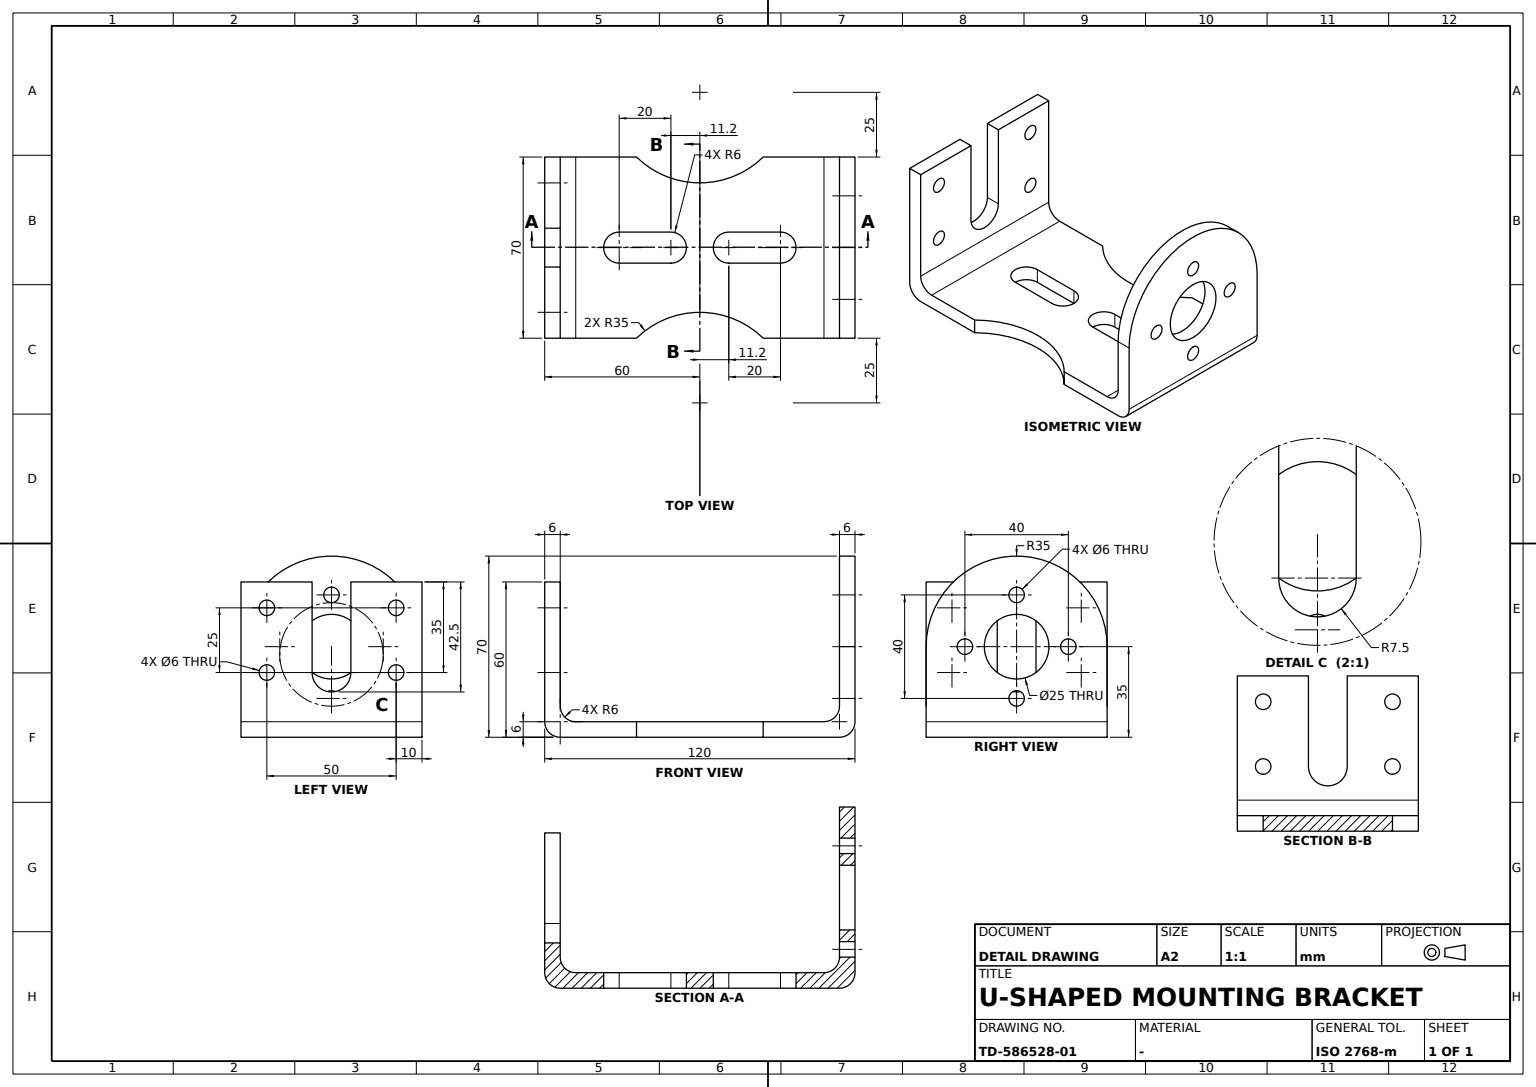
ISO-10303-21;
HEADER;
FILE_DESCRIPTION((''),'2;1');
FILE_NAME('','',(''),(''),'','','');
FILE_SCHEMA(('AUTOMOTIVE_DESIGN'));
ENDSEC;
DATA;
#1=APPLICATION_CONTEXT('');
#2=PRODUCT_CONTEXT('',#1,'mechanical');
#3=PRODUCT('','','',(#2));
#4=PRODUCT_DEFINITION_FORMATION('','',#3);
#5=PRODUCT_DEFINITION_CONTEXT('',#1,'design');
#6=PRODUCT_DEFINITION('','',#4,#5);
#7=PRODUCT_DEFINITION_SHAPE('','',#6);
#8=(LENGTH_UNIT()NAMED_UNIT(*)SI_UNIT(.MILLI.,.METRE.));
#9=(NAMED_UNIT(*)PLANE_ANGLE_UNIT()SI_UNIT($,.RADIAN.));
#10=(NAMED_UNIT(*)SI_UNIT($,.STERADIAN.)SOLID_ANGLE_UNIT());
#11=UNCERTAINTY_MEASURE_WITH_UNIT(LENGTH_MEASURE(0.005),#8,'distance_accuracy_value','');
#12=(GEOMETRIC_REPRESENTATION_CONTEXT(3)GLOBAL_UNCERTAINTY_ASSIGNED_CONTEXT((#11))GLOBAL_UNIT_ASSIGNED_CONTEXT((#8,#9,#10))REPRESENTATION_CONTEXT('',''));
#13=CARTESIAN_POINT('',(70.,35.505103,0.));
#14=VERTEX_POINT('',#13);
#15=CARTESIAN_POINT('',(70.,35.505103,6.));
#16=VERTEX_POINT('',#15);
#17=DIRECTION('',(0.,0.,1.));
#18=VECTOR('',#17,1000.);
#19=LINE('',#13,#18);
#20=EDGE_CURVE('',#14,#16,#19,.T.);
#21=ORIENTED_EDGE('',*,*,#20,.F.);
#22=CARTESIAN_POINT('',(70.,84.494897,0.));
#23=VERTEX_POINT('',#22);
#24=CARTESIAN_POINT('',(95.,60.,0.));
#25=DIRECTION('',(1.,0.,0.));
#26=AXIS2_PLACEMENT_3D('',#24,#17,#25);
#27=CIRCLE('',#26,35.);
#28=EDGE_CURVE('',#23,#14,#27,.T.);
#29=ORIENTED_EDGE('',*,*,#28,.F.);
#30=CARTESIAN_POINT('',(70.,84.494897,6.));
#31=VERTEX_POINT('',#30);
#32=LINE('',#22,#18);
#33=EDGE_CURVE('',#23,#31,#32,.T.);
#34=ORIENTED_EDGE('',*,*,#33,.T.);
#35=CARTESIAN_POINT('',(95.,60.,6.));
#36=AXIS2_PLACEMENT_3D('',#35,#17,#25);
#37=CIRCLE('',#36,35.);
#38=EDGE_CURVE('',#31,#16,#37,.T.);
#39=ORIENTED_EDGE('',*,*,#38,.T.);
#40=EDGE_LOOP('',(#21,#29,#34,#39));
#41=FACE_BOUND('',#40,.T.);
#42=CARTESIAN_POINT('',(95.,60.,3.));
#43=DIRECTION('',(0.,1.,0.));
#44=AXIS2_PLACEMENT_3D('',#42,#17,#43);
#45=CYLINDRICAL_SURFACE('',#44,35.);
#46=ADVANCED_FACE('',(#41),#45,.F.);
#47=CARTESIAN_POINT('',(27.5,6.,25.));
#48=VERTEX_POINT('',#47);
#49=CARTESIAN_POINT('',(42.5,6.,25.));
#50=VERTEX_POINT('',#49);
#51=CARTESIAN_POINT('',(35.,6.,25.));
#52=DIRECTION('',(0.,-1.,0.));
#53=DIRECTION('',(0.,0.,-1.));
#54=AXIS2_PLACEMENT_3D('',#51,#52,#53);
#55=CIRCLE('',#54,7.5);
#56=EDGE_CURVE('',#48,#50,#55,.T.);
#57=ORIENTED_EDGE('',*,*,#56,.F.);
#58=CARTESIAN_POINT('',(27.5,0.,25.));
#59=VERTEX_POINT('',#58);
#60=CARTESIAN_POINT('',(27.5,3.,25.));
#61=VECTOR('',#52,1000.);
#62=LINE('',#60,#61);
#63=EDGE_CURVE('',#59,#48,#62,.F.);
#64=ORIENTED_EDGE('',*,*,#63,.F.);
#65=CARTESIAN_POINT('',(42.5,0.,25.));
#66=VERTEX_POINT('',#65);
#67=CARTESIAN_POINT('',(35.,0.,25.));
#68=AXIS2_PLACEMENT_3D('',#67,#52,#53);
#69=CIRCLE('',#68,7.5);
#70=EDGE_CURVE('',#59,#66,#69,.T.);
#71=ORIENTED_EDGE('',*,*,#70,.T.);
#72=CARTESIAN_POINT('',(42.5,3.,25.));
#73=LINE('',#72,#61);
#74=EDGE_CURVE('',#66,#50,#73,.F.);
#75=ORIENTED_EDGE('',*,*,#74,.T.);
#76=EDGE_LOOP('',(#57,#64,#71,#75));
#77=FACE_BOUND('',#76,.T.);
#78=CARTESIAN_POINT('',(35.,3.,25.));
#79=AXIS2_PLACEMENT_3D('',#78,#52,#25);
#80=CYLINDRICAL_SURFACE('',#79,7.5);
#81=ADVANCED_FACE('',(#77),#80,.F.);
#82=CARTESIAN_POINT('',(70.,6.,0.));
#83=VERTEX_POINT('',#82);
#84=CARTESIAN_POINT('',(70.,0.,0.));
#85=LINE('',#84,#61);
#86=EDGE_CURVE('',#14,#83,#85,.T.);
#87=ORIENTED_EDGE('',*,*,#86,.F.);
#88=ORIENTED_EDGE('',*,*,#20,.T.);
#89=CARTESIAN_POINT('',(70.,12.,6.));
#90=VERTEX_POINT('',#89);
#91=CARTESIAN_POINT('',(70.,0.,6.));
#92=LINE('',#91,#61);
#93=EDGE_CURVE('',#16,#90,#92,.T.);
#94=ORIENTED_EDGE('',*,*,#93,.T.);
#95=CARTESIAN_POINT('',(70.,6.,12.));
#96=VERTEX_POINT('',#95);
#97=CARTESIAN_POINT('',(70.,12.,12.));
#98=DIRECTION('',(-1.,0.,0.));
#99=AXIS2_PLACEMENT_3D('',#97,#98,#17);
#100=CIRCLE('',#99,6.);
#101=EDGE_CURVE('',#90,#96,#100,.T.);
#102=ORIENTED_EDGE('',*,*,#101,.T.);
#103=CARTESIAN_POINT('',(70.,6.,60.));
#104=VERTEX_POINT('',#103);
#105=LINE('',#82,#18);
#106=EDGE_CURVE('',#96,#104,#105,.T.);
#107=ORIENTED_EDGE('',*,*,#106,.T.);
#108=CARTESIAN_POINT('',(70.,0.,60.));
#109=VERTEX_POINT('',#108);
#110=VECTOR('',#43,1000.);
#111=LINE('',#108,#110);
#112=EDGE_CURVE('',#109,#104,#111,.T.);
#113=ORIENTED_EDGE('',*,*,#112,.F.);
#114=VERTEX_POINT('',#91);
#115=LINE('',#84,#18);
#116=EDGE_CURVE('',#114,#109,#115,.T.);
#117=ORIENTED_EDGE('',*,*,#116,.F.);
#118=CARTESIAN_POINT('',(70.,6.,6.));
#119=AXIS2_PLACEMENT_3D('',#118,#98,#17);
#120=CIRCLE('',#119,6.);
#121=EDGE_CURVE('',#83,#114,#120,.T.);
#122=ORIENTED_EDGE('',*,*,#121,.F.);
#123=EDGE_LOOP('',(#87,#88,#94,#102,#107,#113,#117,#122));
#124=FACE_BOUND('',#123,.T.);
#125=AXIS2_PLACEMENT_3D('',#13,#98,#52);
#126=PLANE('',#125);
#127=ADVANCED_FACE('',(#124),#126,.F.);
#128=CARTESIAN_POINT('',(41.,48.80349,0.));
#129=VERTEX_POINT('',#128);
#130=CARTESIAN_POINT('',(41.,28.80349,0.));
#131=VERTEX_POINT('',#130);
#132=LINE('',#128,#61);
#133=EDGE_CURVE('',#129,#131,#132,.T.);
#134=ORIENTED_EDGE('',*,*,#133,.T.);
#135=CARTESIAN_POINT('',(41.,28.80349,6.));
#136=VERTEX_POINT('',#135);
#137=CARTESIAN_POINT('',(41.,28.80349,2.34));
#138=LINE('',#137,#18);
#139=EDGE_CURVE('',#136,#131,#138,.F.);
#140=ORIENTED_EDGE('',*,*,#139,.F.);
#141=CARTESIAN_POINT('',(41.,48.80349,6.));
#142=VERTEX_POINT('',#141);
#143=LINE('',#141,#61);
#144=EDGE_CURVE('',#142,#136,#143,.T.);
#145=ORIENTED_EDGE('',*,*,#144,.F.);
#146=CARTESIAN_POINT('',(41.,48.80349,2.34));
#147=LINE('',#146,#18);
#148=EDGE_CURVE('',#142,#129,#147,.F.);
#149=ORIENTED_EDGE('',*,*,#148,.T.);
#150=EDGE_LOOP('',(#134,#140,#145,#149));
#151=FACE_BOUND('',#150,.T.);
#152=AXIS2_PLACEMENT_3D('',#141,#25,#52);
#153=PLANE('',#152);
#154=ADVANCED_FACE('',(#151),#153,.F.);
#155=CARTESIAN_POINT('',(29.,71.19651,0.));
#156=VERTEX_POINT('',#155);
#157=CARTESIAN_POINT('',(29.,91.19651,0.));
#158=VERTEX_POINT('',#157);
#159=CARTESIAN_POINT('',(29.,28.80349,0.));
#160=LINE('',#159,#110);
#161=EDGE_CURVE('',#156,#158,#160,.T.);
#162=ORIENTED_EDGE('',*,*,#161,.T.);
#163=CARTESIAN_POINT('',(29.,91.19651,6.));
#164=VERTEX_POINT('',#163);
#165=CARTESIAN_POINT('',(29.,91.19651,2.34));
#166=LINE('',#165,#18);
#167=EDGE_CURVE('',#164,#158,#166,.F.);
#168=ORIENTED_EDGE('',*,*,#167,.F.);
#169=CARTESIAN_POINT('',(29.,71.19651,6.));
#170=VERTEX_POINT('',#169);
#171=CARTESIAN_POINT('',(29.,0.,6.));
#172=LINE('',#171,#61);
#173=EDGE_CURVE('',#164,#170,#172,.T.);
#174=ORIENTED_EDGE('',*,*,#173,.T.);
#175=CARTESIAN_POINT('',(29.,71.19651,2.34));
#176=LINE('',#175,#18);
#177=EDGE_CURVE('',#170,#156,#176,.F.);
#178=ORIENTED_EDGE('',*,*,#177,.T.);
#179=EDGE_LOOP('',(#162,#168,#174,#178));
#180=FACE_BOUND('',#179,.T.);
#181=CARTESIAN_POINT('',(29.,28.80349,6.));
#182=AXIS2_PLACEMENT_3D('',#181,#98,#43);
#183=PLANE('',#182);
#184=ADVANCED_FACE('',(#180),#183,.F.);
#185=ORIENTED_EDGE('',*,*,#177,.F.);
#186=CARTESIAN_POINT('',(41.,71.19651,6.));
#187=VERTEX_POINT('',#186);
#188=CARTESIAN_POINT('',(35.,71.19651,6.));
#189=AXIS2_PLACEMENT_3D('',#188,#17,#25);
#190=CIRCLE('',#189,6.);
#191=EDGE_CURVE('',#170,#187,#190,.T.);
#192=ORIENTED_EDGE('',*,*,#191,.T.);
#193=CARTESIAN_POINT('',(41.,71.19651,0.));
#194=VERTEX_POINT('',#193);
#195=CARTESIAN_POINT('',(41.,71.19651,2.34));
#196=LINE('',#195,#18);
#197=EDGE_CURVE('',#187,#194,#196,.F.);
#198=ORIENTED_EDGE('',*,*,#197,.T.);
#199=CARTESIAN_POINT('',(35.,71.19651,0.));
#200=AXIS2_PLACEMENT_3D('',#199,#17,#25);
#201=CIRCLE('',#200,6.);
#202=EDGE_CURVE('',#156,#194,#201,.T.);
#203=ORIENTED_EDGE('',*,*,#202,.F.);
#204=EDGE_LOOP('',(#185,#192,#198,#203));
#205=FACE_BOUND('',#204,.T.);
#206=CARTESIAN_POINT('',(35.,71.19651,2.34));
#207=AXIS2_PLACEMENT_3D('',#206,#17,#43);
#208=CYLINDRICAL_SURFACE('',#207,6.);
#209=ADVANCED_FACE('',(#205),#208,.F.);
#210=CARTESIAN_POINT('',(35.,114.,12.));
#211=VERTEX_POINT('',#210);
#212=CARTESIAN_POINT('',(70.,114.,12.));
#213=VERTEX_POINT('',#212);
#214=VECTOR('',#25,1000.);
#215=LINE('',#210,#214);
#216=EDGE_CURVE('',#211,#213,#215,.T.);
#217=ORIENTED_EDGE('',*,*,#216,.F.);
#218=CARTESIAN_POINT('',(0.,114.,12.));
#219=VERTEX_POINT('',#218);
#220=EDGE_CURVE('',#219,#211,#215,.T.);
#221=ORIENTED_EDGE('',*,*,#220,.F.);
#222=CARTESIAN_POINT('',(0.,108.,6.));
#223=VERTEX_POINT('',#222);
#224=CARTESIAN_POINT('',(0.,108.,12.));
#225=AXIS2_PLACEMENT_3D('',#224,#25,#53);
#226=CIRCLE('',#225,6.);
#227=EDGE_CURVE('',#223,#219,#226,.T.);
#228=ORIENTED_EDGE('',*,*,#227,.F.);
#229=CARTESIAN_POINT('',(70.,108.,6.));
#230=VERTEX_POINT('',#229);
#231=CARTESIAN_POINT('',(35.,108.,6.));
#232=LINE('',#231,#214);
#233=EDGE_CURVE('',#223,#230,#232,.T.);
#234=ORIENTED_EDGE('',*,*,#233,.T.);
#235=CARTESIAN_POINT('',(70.,108.,12.));
#236=AXIS2_PLACEMENT_3D('',#235,#98,#17);
#237=CIRCLE('',#236,6.);
#238=EDGE_CURVE('',#213,#230,#237,.T.);
#239=ORIENTED_EDGE('',*,*,#238,.F.);
#240=EDGE_LOOP('',(#217,#221,#228,#234,#239));
#241=FACE_BOUND('',#240,.T.);
#242=CARTESIAN_POINT('',(35.,108.,12.));
#243=AXIS2_PLACEMENT_3D('',#242,#25,#53);
#244=CYLINDRICAL_SURFACE('',#243,6.);
#245=ADVANCED_FACE('',(#241),#244,.F.);
#246=CARTESIAN_POINT('',(0.,0.,60.));
#247=VERTEX_POINT('',#246);
#248=CARTESIAN_POINT('',(0.,6.,60.));
#249=VERTEX_POINT('',#248);
#250=CARTESIAN_POINT('',(0.,84.494897,60.));
#251=LINE('',#250,#110);
#252=EDGE_CURVE('',#247,#249,#251,.T.);
#253=ORIENTED_EDGE('',*,*,#252,.F.);
#254=CARTESIAN_POINT('',(27.5,0.,60.));
#255=VERTEX_POINT('',#254);
#256=VECTOR('',#98,1000.);
#257=LINE('',#108,#256);
#258=EDGE_CURVE('',#255,#247,#257,.T.);
#259=ORIENTED_EDGE('',*,*,#258,.F.);
#260=CARTESIAN_POINT('',(27.5,6.,60.));
#261=VERTEX_POINT('',#260);
#262=LINE('',#254,#61);
#263=EDGE_CURVE('',#261,#255,#262,.T.);
#264=ORIENTED_EDGE('',*,*,#263,.F.);
#265=LINE('',#103,#256);
#266=EDGE_CURVE('',#261,#249,#265,.T.);
#267=ORIENTED_EDGE('',*,*,#266,.T.);
#268=EDGE_LOOP('',(#253,#259,#264,#267));
#269=FACE_BOUND('',#268,.T.);
#270=AXIS2_PLACEMENT_3D('',#108,#53,#98);
#271=PLANE('',#270);
#272=ADVANCED_FACE('',(#269),#271,.F.);
#273=CARTESIAN_POINT('',(35.,120.,18.));
#274=VERTEX_POINT('',#273);
#275=CARTESIAN_POINT('',(35.,120.,15.));
#276=AXIS2_PLACEMENT_3D('',#275,#43,#17);
#277=CIRCLE('',#276,3.);
#278=EDGE_CURVE('',#274,#274,#277,.T.);
#279=ORIENTED_EDGE('',*,*,#278,.T.);
#280=EDGE_LOOP('',(#279));
#281=FACE_BOUND('',#280,.T.);
#282=CARTESIAN_POINT('',(35.,114.,15.));
#283=AXIS2_PLACEMENT_3D('',#282,#43,#17);
#284=CIRCLE('',#283,3.);
#285=EDGE_CURVE('',#211,#211,#284,.T.);
#286=ORIENTED_EDGE('',*,*,#285,.F.);
#287=EDGE_LOOP('',(#286));
#288=FACE_BOUND('',#287,.T.);
#289=CARTESIAN_POINT('',(35.,59.34,15.));
#290=AXIS2_PLACEMENT_3D('',#289,#43,#98);
#291=CYLINDRICAL_SURFACE('',#290,3.);
#292=ADVANCED_FACE('',(#281,#288),#291,.F.);
#293=CARTESIAN_POINT('',(70.,114.,0.));
#294=VERTEX_POINT('',#293);
#295=EDGE_CURVE('',#294,#23,#85,.T.);
#296=ORIENTED_EDGE('',*,*,#295,.F.);
#297=CARTESIAN_POINT('',(70.,120.,6.));
#298=VERTEX_POINT('',#297);
#299=CARTESIAN_POINT('',(70.,114.,6.));
#300=AXIS2_PLACEMENT_3D('',#299,#98,#17);
#301=CIRCLE('',#300,6.);
#302=EDGE_CURVE('',#298,#294,#301,.T.);
#303=ORIENTED_EDGE('',*,*,#302,.F.);
#304=CARTESIAN_POINT('',(70.,120.,35.));
#305=VERTEX_POINT('',#304);
#306=CARTESIAN_POINT('',(70.,120.,0.));
#307=LINE('',#306,#18);
#308=EDGE_CURVE('',#298,#305,#307,.T.);
#309=ORIENTED_EDGE('',*,*,#308,.T.);
#310=CARTESIAN_POINT('',(70.,114.,35.));
#311=VERTEX_POINT('',#310);
#312=CARTESIAN_POINT('',(70.,117.,35.));
#313=LINE('',#312,#110);
#314=EDGE_CURVE('',#305,#311,#313,.F.);
#315=ORIENTED_EDGE('',*,*,#314,.T.);
#316=LINE('',#293,#18);
#317=EDGE_CURVE('',#213,#311,#316,.T.);
#318=ORIENTED_EDGE('',*,*,#317,.F.);
#319=ORIENTED_EDGE('',*,*,#238,.T.);
#320=EDGE_CURVE('',#230,#31,#92,.T.);
#321=ORIENTED_EDGE('',*,*,#320,.T.);
#322=ORIENTED_EDGE('',*,*,#33,.F.);
#323=EDGE_LOOP('',(#296,#303,#309,#315,#318,#319,#321,#322));
#324=FACE_BOUND('',#323,.T.);
#325=ADVANCED_FACE('',(#324),#126,.F.);
#326=CARTESIAN_POINT('',(60.,6.,22.));
#327=VERTEX_POINT('',#326);
#328=CARTESIAN_POINT('',(60.,6.,25.));
#329=AXIS2_PLACEMENT_3D('',#328,#52,#53);
#330=CIRCLE('',#329,3.);
#331=EDGE_CURVE('',#327,#327,#330,.T.);
#332=ORIENTED_EDGE('',*,*,#331,.F.);
#333=EDGE_LOOP('',(#332));
#334=FACE_BOUND('',#333,.T.);
#335=CARTESIAN_POINT('',(60.,0.,22.));
#336=VERTEX_POINT('',#335);
#337=CARTESIAN_POINT('',(60.,0.,25.));
#338=AXIS2_PLACEMENT_3D('',#337,#52,#53);
#339=CIRCLE('',#338,3.);
#340=EDGE_CURVE('',#336,#336,#339,.T.);
#341=ORIENTED_EDGE('',*,*,#340,.T.);
#342=EDGE_LOOP('',(#341));
#343=FACE_BOUND('',#342,.T.);
#344=CARTESIAN_POINT('',(60.,60.66,25.));
#345=AXIS2_PLACEMENT_3D('',#344,#52,#25);
#346=CYLINDRICAL_SURFACE('',#345,3.);
#347=ADVANCED_FACE('',(#334,#343),#346,.F.);
#348=CARTESIAN_POINT('',(15.,114.,38.));
#349=VERTEX_POINT('',#348);
#350=CARTESIAN_POINT('',(15.,114.,35.));
#351=AXIS2_PLACEMENT_3D('',#350,#43,#17);
#352=CIRCLE('',#351,3.);
#353=EDGE_CURVE('',#349,#349,#352,.T.);
#354=ORIENTED_EDGE('',*,*,#353,.F.);
#355=EDGE_LOOP('',(#354));
#356=FACE_BOUND('',#355,.T.);
#357=CARTESIAN_POINT('',(15.,120.,38.));
#358=VERTEX_POINT('',#357);
#359=CARTESIAN_POINT('',(15.,120.,35.));
#360=AXIS2_PLACEMENT_3D('',#359,#43,#17);
#361=CIRCLE('',#360,3.);
#362=EDGE_CURVE('',#358,#358,#361,.T.);
#363=ORIENTED_EDGE('',*,*,#362,.T.);
#364=EDGE_LOOP('',(#363));
#365=FACE_BOUND('',#364,.T.);
#366=CARTESIAN_POINT('',(15.,59.34,35.));
#367=AXIS2_PLACEMENT_3D('',#366,#43,#98);
#368=CYLINDRICAL_SURFACE('',#367,3.);
#369=ADVANCED_FACE('',(#356,#365),#368,.F.);
#370=ORIENTED_EDGE('',*,*,#101,.F.);
#371=CARTESIAN_POINT('',(0.,12.,6.));
#372=VERTEX_POINT('',#371);
#373=CARTESIAN_POINT('',(35.,12.,6.));
#374=LINE('',#373,#214);
#375=EDGE_CURVE('',#372,#90,#374,.T.);
#376=ORIENTED_EDGE('',*,*,#375,.F.);
#377=CARTESIAN_POINT('',(0.,6.,12.));
#378=VERTEX_POINT('',#377);
#379=CARTESIAN_POINT('',(0.,12.,12.));
#380=AXIS2_PLACEMENT_3D('',#379,#25,#53);
#381=CIRCLE('',#380,6.);
#382=EDGE_CURVE('',#378,#372,#381,.T.);
#383=ORIENTED_EDGE('',*,*,#382,.F.);
#384=CARTESIAN_POINT('',(35.,6.,12.));
#385=LINE('',#384,#214);
#386=EDGE_CURVE('',#378,#96,#385,.T.);
#387=ORIENTED_EDGE('',*,*,#386,.T.);
#388=EDGE_LOOP('',(#370,#376,#383,#387));
#389=FACE_BOUND('',#388,.T.);
#390=CARTESIAN_POINT('',(35.,12.,12.));
#391=AXIS2_PLACEMENT_3D('',#390,#25,#52);
#392=CYLINDRICAL_SURFACE('',#391,6.);
#393=ADVANCED_FACE('',(#389),#392,.F.);
#394=CARTESIAN_POINT('',(10.,6.,47.));
#395=VERTEX_POINT('',#394);
#396=CARTESIAN_POINT('',(10.,6.,50.));
#397=AXIS2_PLACEMENT_3D('',#396,#52,#53);
#398=CIRCLE('',#397,3.);
#399=EDGE_CURVE('',#395,#395,#398,.T.);
#400=ORIENTED_EDGE('',*,*,#399,.F.);
#401=EDGE_LOOP('',(#400));
#402=FACE_BOUND('',#401,.T.);
#403=CARTESIAN_POINT('',(10.,0.,47.));
#404=VERTEX_POINT('',#403);
#405=CARTESIAN_POINT('',(10.,0.,50.));
#406=AXIS2_PLACEMENT_3D('',#405,#52,#53);
#407=CIRCLE('',#406,3.);
#408=EDGE_CURVE('',#404,#404,#407,.T.);
#409=ORIENTED_EDGE('',*,*,#408,.T.);
#410=EDGE_LOOP('',(#409));
#411=FACE_BOUND('',#410,.T.);
#412=CARTESIAN_POINT('',(10.,60.66,50.));
#413=AXIS2_PLACEMENT_3D('',#412,#52,#25);
#414=CYLINDRICAL_SURFACE('',#413,3.);
#415=ADVANCED_FACE('',(#402,#411),#414,.F.);
#416=CARTESIAN_POINT('',(0.,0.,6.));
#417=VERTEX_POINT('',#416);
#418=CARTESIAN_POINT('',(0.,6.,0.));
#419=VERTEX_POINT('',#418);
#420=CARTESIAN_POINT('',(0.,6.,6.));
#421=AXIS2_PLACEMENT_3D('',#420,#25,#53);
#422=CIRCLE('',#421,6.);
#423=EDGE_CURVE('',#417,#419,#422,.T.);
#424=ORIENTED_EDGE('',*,*,#423,.F.);
#425=CARTESIAN_POINT('',(0.,0.,0.));
#426=VECTOR('',#53,1000.);
#427=LINE('',#425,#426);
#428=EDGE_CURVE('',#247,#417,#427,.T.);
#429=ORIENTED_EDGE('',*,*,#428,.F.);
#430=ORIENTED_EDGE('',*,*,#252,.T.);
#431=LINE('',#418,#426);
#432=EDGE_CURVE('',#249,#378,#431,.T.);
#433=ORIENTED_EDGE('',*,*,#432,.T.);
#434=ORIENTED_EDGE('',*,*,#382,.T.);
#435=CARTESIAN_POINT('',(0.,35.505103,6.));
#436=VERTEX_POINT('',#435);
#437=LINE('',#416,#110);
#438=EDGE_CURVE('',#372,#436,#437,.T.);
#439=ORIENTED_EDGE('',*,*,#438,.T.);
#440=CARTESIAN_POINT('',(0.,35.505103,0.));
#441=VERTEX_POINT('',#440);
#442=LINE('',#440,#18);
#443=EDGE_CURVE('',#441,#436,#442,.T.);
#444=ORIENTED_EDGE('',*,*,#443,.F.);
#445=LINE('',#425,#110);
#446=EDGE_CURVE('',#419,#441,#445,.T.);
#447=ORIENTED_EDGE('',*,*,#446,.F.);
#448=EDGE_LOOP('',(#424,#429,#430,#433,#434,#439,#444,#447));
#449=FACE_BOUND('',#448,.T.);
#450=CARTESIAN_POINT('',(0.,84.494897,0.));
#451=AXIS2_PLACEMENT_3D('',#450,#25,#43);
#452=PLANE('',#451);
#453=ADVANCED_FACE('',(#449),#452,.F.);
#454=CARTESIAN_POINT('',(29.,48.80349,0.));
#455=VERTEX_POINT('',#454);
#456=CARTESIAN_POINT('',(35.,48.80349,0.));
#457=AXIS2_PLACEMENT_3D('',#456,#17,#25);
#458=CIRCLE('',#457,6.);
#459=EDGE_CURVE('',#129,#455,#458,.T.);
#460=ORIENTED_EDGE('',*,*,#459,.F.);
#461=ORIENTED_EDGE('',*,*,#148,.F.);
#462=CARTESIAN_POINT('',(29.,48.80349,6.));
#463=VERTEX_POINT('',#462);
#464=CARTESIAN_POINT('',(35.,48.80349,6.));
#465=AXIS2_PLACEMENT_3D('',#464,#17,#25);
#466=CIRCLE('',#465,6.);
#467=EDGE_CURVE('',#142,#463,#466,.T.);
#468=ORIENTED_EDGE('',*,*,#467,.T.);
#469=CARTESIAN_POINT('',(29.,48.80349,2.34));
#470=LINE('',#469,#18);
#471=EDGE_CURVE('',#463,#455,#470,.F.);
#472=ORIENTED_EDGE('',*,*,#471,.T.);
#473=EDGE_LOOP('',(#460,#461,#468,#472));
#474=FACE_BOUND('',#473,.T.);
#475=CARTESIAN_POINT('',(35.,48.80349,2.34));
#476=AXIS2_PLACEMENT_3D('',#475,#17,#43);
#477=CYLINDRICAL_SURFACE('',#476,6.);
#478=ADVANCED_FACE('',(#474),#477,.F.);
#479=VERTEX_POINT('',#450);
#480=CARTESIAN_POINT('',(0.,84.494897,6.));
#481=VERTEX_POINT('',#480);
#482=LINE('',#450,#18);
#483=EDGE_CURVE('',#479,#481,#482,.T.);
#484=ORIENTED_EDGE('',*,*,#483,.T.);
#485=EDGE_CURVE('',#481,#223,#437,.T.);
#486=ORIENTED_EDGE('',*,*,#485,.T.);
#487=ORIENTED_EDGE('',*,*,#227,.T.);
#488=CARTESIAN_POINT('',(0.,114.,35.));
#489=VERTEX_POINT('',#488);
#490=CARTESIAN_POINT('',(0.,114.,0.));
#491=LINE('',#490,#18);
#492=EDGE_CURVE('',#219,#489,#491,.T.);
#493=ORIENTED_EDGE('',*,*,#492,.T.);
#494=CARTESIAN_POINT('',(0.,120.,35.));
#495=VERTEX_POINT('',#494);
#496=CARTESIAN_POINT('',(0.,117.,35.));
#497=LINE('',#496,#110);
#498=EDGE_CURVE('',#495,#489,#497,.F.);
#499=ORIENTED_EDGE('',*,*,#498,.F.);
#500=CARTESIAN_POINT('',(0.,120.,6.));
#501=VERTEX_POINT('',#500);
#502=CARTESIAN_POINT('',(0.,120.,0.));
#503=LINE('',#502,#18);
#504=EDGE_CURVE('',#501,#495,#503,.T.);
#505=ORIENTED_EDGE('',*,*,#504,.F.);
#506=VERTEX_POINT('',#490);
#507=CARTESIAN_POINT('',(0.,114.,6.));
#508=AXIS2_PLACEMENT_3D('',#507,#25,#53);
#509=CIRCLE('',#508,6.);
#510=EDGE_CURVE('',#506,#501,#509,.T.);
#511=ORIENTED_EDGE('',*,*,#510,.F.);
#512=EDGE_CURVE('',#479,#506,#445,.T.);
#513=ORIENTED_EDGE('',*,*,#512,.F.);
#514=EDGE_LOOP('',(#484,#486,#487,#493,#499,#505,#511,#513));
#515=FACE_BOUND('',#514,.T.);
#516=ADVANCED_FACE('',(#515),#452,.F.);
#517=CARTESIAN_POINT('',(41.,91.19651,0.));
#518=VERTEX_POINT('',#517);
#519=CARTESIAN_POINT('',(35.,91.19651,0.));
#520=AXIS2_PLACEMENT_3D('',#519,#17,#25);
#521=CIRCLE('',#520,6.);
#522=EDGE_CURVE('',#518,#158,#521,.T.);
#523=ORIENTED_EDGE('',*,*,#522,.T.);
#524=ORIENTED_EDGE('',*,*,#161,.F.);
#525=ORIENTED_EDGE('',*,*,#202,.T.);
#526=EDGE_CURVE('',#518,#194,#132,.T.);
#527=ORIENTED_EDGE('',*,*,#526,.F.);
#528=EDGE_LOOP('',(#523,#524,#525,#527));
#529=FACE_BOUND('',#528,.T.);
#530=ORIENTED_EDGE('',*,*,#512,.T.);
#531=CARTESIAN_POINT('',(35.,114.,0.));
#532=LINE('',#531,#256);
#533=EDGE_CURVE('',#294,#506,#532,.T.);
#534=ORIENTED_EDGE('',*,*,#533,.F.);
#535=ORIENTED_EDGE('',*,*,#295,.T.);
#536=ORIENTED_EDGE('',*,*,#28,.T.);
#537=ORIENTED_EDGE('',*,*,#86,.T.);
#538=CARTESIAN_POINT('',(35.,6.,0.));
#539=LINE('',#538,#214);
#540=EDGE_CURVE('',#419,#83,#539,.T.);
#541=ORIENTED_EDGE('',*,*,#540,.F.);
#542=ORIENTED_EDGE('',*,*,#446,.T.);
#543=CARTESIAN_POINT('',(-25.,60.,0.));
#544=AXIS2_PLACEMENT_3D('',#543,#17,#25);
#545=CIRCLE('',#544,35.);
#546=EDGE_CURVE('',#441,#479,#545,.T.);
#547=ORIENTED_EDGE('',*,*,#546,.T.);
#548=EDGE_LOOP('',(#530,#534,#535,#536,#537,#541,#542,#547));
#549=FACE_BOUND('',#548,.T.);
#550=VERTEX_POINT('',#159);
#551=EDGE_CURVE('',#550,#455,#160,.T.);
#552=ORIENTED_EDGE('',*,*,#551,.F.);
#553=CARTESIAN_POINT('',(35.,28.80349,0.));
#554=AXIS2_PLACEMENT_3D('',#553,#17,#25);
#555=CIRCLE('',#554,6.);
#556=EDGE_CURVE('',#550,#131,#555,.T.);
#557=ORIENTED_EDGE('',*,*,#556,.T.);
#558=ORIENTED_EDGE('',*,*,#133,.F.);
#559=ORIENTED_EDGE('',*,*,#459,.T.);
#560=EDGE_LOOP('',(#552,#557,#558,#559));
#561=FACE_BOUND('',#560,.T.);
#562=AXIS2_PLACEMENT_3D('',#425,#17,#43);
#563=PLANE('',#562);
#564=ADVANCED_FACE('',(#529,#549,#561),#563,.F.);
#565=ORIENTED_EDGE('',*,*,#483,.F.);
#566=ORIENTED_EDGE('',*,*,#546,.F.);
#567=ORIENTED_EDGE('',*,*,#443,.T.);
#568=CARTESIAN_POINT('',(-25.,60.,6.));
#569=AXIS2_PLACEMENT_3D('',#568,#17,#25);
#570=CIRCLE('',#569,35.);
#571=EDGE_CURVE('',#436,#481,#570,.T.);
#572=ORIENTED_EDGE('',*,*,#571,.T.);
#573=EDGE_LOOP('',(#565,#566,#567,#572));
#574=FACE_BOUND('',#573,.T.);
#575=CARTESIAN_POINT('',(-25.,60.,3.));
#576=AXIS2_PLACEMENT_3D('',#575,#17,#43);
#577=CYLINDRICAL_SURFACE('',#576,35.);
#578=ADVANCED_FACE('',(#574),#577,.F.);
#579=ORIENTED_EDGE('',*,*,#112,.T.);
#580=CARTESIAN_POINT('',(42.5,6.,60.));
#581=VERTEX_POINT('',#580);
#582=EDGE_CURVE('',#104,#581,#265,.T.);
#583=ORIENTED_EDGE('',*,*,#582,.T.);
#584=CARTESIAN_POINT('',(42.5,0.,60.));
#585=VERTEX_POINT('',#584);
#586=LINE('',#584,#61);
#587=EDGE_CURVE('',#581,#585,#586,.T.);
#588=ORIENTED_EDGE('',*,*,#587,.T.);
#589=EDGE_CURVE('',#109,#585,#257,.T.);
#590=ORIENTED_EDGE('',*,*,#589,.F.);
#591=EDGE_LOOP('',(#579,#583,#588,#590));
#592=FACE_BOUND('',#591,.T.);
#593=ADVANCED_FACE('',(#592),#271,.F.);
#594=CARTESIAN_POINT('',(55.,120.,38.));
#595=VERTEX_POINT('',#594);
#596=CARTESIAN_POINT('',(55.,120.,35.));
#597=AXIS2_PLACEMENT_3D('',#596,#43,#17);
#598=CIRCLE('',#597,3.);
#599=EDGE_CURVE('',#595,#595,#598,.T.);
#600=ORIENTED_EDGE('',*,*,#599,.T.);
#601=EDGE_LOOP('',(#600));
#602=FACE_BOUND('',#601,.T.);
#603=CARTESIAN_POINT('',(55.,114.,38.));
#604=VERTEX_POINT('',#603);
#605=CARTESIAN_POINT('',(55.,114.,35.));
#606=AXIS2_PLACEMENT_3D('',#605,#43,#17);
#607=CIRCLE('',#606,3.);
#608=EDGE_CURVE('',#604,#604,#607,.T.);
#609=ORIENTED_EDGE('',*,*,#608,.F.);
#610=EDGE_LOOP('',(#609));
#611=FACE_BOUND('',#610,.T.);
#612=CARTESIAN_POINT('',(55.,59.34,35.));
#613=AXIS2_PLACEMENT_3D('',#612,#43,#98);
#614=CYLINDRICAL_SURFACE('',#613,3.);
#615=ADVANCED_FACE('',(#602,#611),#614,.F.);
#616=CARTESIAN_POINT('',(35.,114.,58.));
#617=VERTEX_POINT('',#616);
#618=CARTESIAN_POINT('',(35.,114.,55.));
#619=AXIS2_PLACEMENT_3D('',#618,#43,#17);
#620=CIRCLE('',#619,3.);
#621=EDGE_CURVE('',#617,#617,#620,.T.);
#622=ORIENTED_EDGE('',*,*,#621,.F.);
#623=EDGE_LOOP('',(#622));
#624=FACE_BOUND('',#623,.T.);
#625=CARTESIAN_POINT('',(35.,120.,58.));
#626=VERTEX_POINT('',#625);
#627=CARTESIAN_POINT('',(35.,120.,55.));
#628=AXIS2_PLACEMENT_3D('',#627,#43,#17);
#629=CIRCLE('',#628,3.);
#630=EDGE_CURVE('',#626,#626,#629,.T.);
#631=ORIENTED_EDGE('',*,*,#630,.T.);
#632=EDGE_LOOP('',(#631));
#633=FACE_BOUND('',#632,.T.);
#634=CARTESIAN_POINT('',(35.,59.34,55.));
#635=AXIS2_PLACEMENT_3D('',#634,#43,#98);
#636=CYLINDRICAL_SURFACE('',#635,3.);
#637=ADVANCED_FACE('',(#624,#633),#636,.F.);
#638=CARTESIAN_POINT('',(41.,91.19651,6.));
#639=VERTEX_POINT('',#638);
#640=CARTESIAN_POINT('',(41.,91.19651,2.34));
#641=LINE('',#640,#18);
#642=EDGE_CURVE('',#639,#518,#641,.F.);
#643=ORIENTED_EDGE('',*,*,#642,.F.);
#644=CARTESIAN_POINT('',(35.,91.19651,6.));
#645=AXIS2_PLACEMENT_3D('',#644,#17,#25);
#646=CIRCLE('',#645,6.);
#647=EDGE_CURVE('',#639,#164,#646,.T.);
#648=ORIENTED_EDGE('',*,*,#647,.T.);
#649=ORIENTED_EDGE('',*,*,#167,.T.);
#650=ORIENTED_EDGE('',*,*,#522,.F.);
#651=EDGE_LOOP('',(#643,#648,#649,#650));
#652=FACE_BOUND('',#651,.T.);
#653=CARTESIAN_POINT('',(35.,91.19651,2.34));
#654=AXIS2_PLACEMENT_3D('',#653,#17,#43);
#655=CYLINDRICAL_SURFACE('',#654,6.);
#656=ADVANCED_FACE('',(#652),#655,.F.);
#657=ORIENTED_EDGE('',*,*,#302,.T.);
#658=ORIENTED_EDGE('',*,*,#533,.T.);
#659=ORIENTED_EDGE('',*,*,#510,.T.);
#660=CARTESIAN_POINT('',(35.,120.,6.));
#661=LINE('',#660,#256);
#662=EDGE_CURVE('',#298,#501,#661,.T.);
#663=ORIENTED_EDGE('',*,*,#662,.F.);
#664=EDGE_LOOP('',(#657,#658,#659,#663));
#665=FACE_BOUND('',#664,.T.);
#666=CARTESIAN_POINT('',(35.,114.,6.));
#667=AXIS2_PLACEMENT_3D('',#666,#98,#53);
#668=CYLINDRICAL_SURFACE('',#667,6.);
#669=ADVANCED_FACE('',(#665),#668,.T.);
#670=CARTESIAN_POINT('',(35.,0.,6.));
#671=LINE('',#670,#214);
#672=EDGE_CURVE('',#417,#114,#671,.T.);
#673=ORIENTED_EDGE('',*,*,#672,.F.);
#674=ORIENTED_EDGE('',*,*,#423,.T.);
#675=ORIENTED_EDGE('',*,*,#540,.T.);
#676=ORIENTED_EDGE('',*,*,#121,.T.);
#677=EDGE_LOOP('',(#673,#674,#675,#676));
#678=FACE_BOUND('',#677,.T.);
#679=CARTESIAN_POINT('',(35.,6.,6.));
#680=AXIS2_PLACEMENT_3D('',#679,#25,#53);
#681=CYLINDRICAL_SURFACE('',#680,6.);
#682=ADVANCED_FACE('',(#678),#681,.T.);
#683=ORIENTED_EDGE('',*,*,#63,.T.);
#684=LINE('',#47,#18);
#685=EDGE_CURVE('',#48,#261,#684,.T.);
#686=ORIENTED_EDGE('',*,*,#685,.T.);
#687=ORIENTED_EDGE('',*,*,#263,.T.);
#688=LINE('',#58,#18);
#689=EDGE_CURVE('',#59,#255,#688,.T.);
#690=ORIENTED_EDGE('',*,*,#689,.F.);
#691=EDGE_LOOP('',(#683,#686,#687,#690));
#692=FACE_BOUND('',#691,.T.);
#693=AXIS2_PLACEMENT_3D('',#58,#98,#17);
#694=PLANE('',#693);
#695=ADVANCED_FACE('',(#692),#694,.F.);
#696=CARTESIAN_POINT('',(60.,6.,47.));
#697=VERTEX_POINT('',#696);
#698=CARTESIAN_POINT('',(60.,6.,50.));
#699=AXIS2_PLACEMENT_3D('',#698,#52,#53);
#700=CIRCLE('',#699,3.);
#701=EDGE_CURVE('',#697,#697,#700,.T.);
#702=ORIENTED_EDGE('',*,*,#701,.T.);
#703=EDGE_LOOP('',(#702));
#704=FACE_BOUND('',#703,.T.);
#705=CARTESIAN_POINT('',(10.,6.,22.));
#706=VERTEX_POINT('',#705);
#707=CARTESIAN_POINT('',(10.,6.,25.));
#708=AXIS2_PLACEMENT_3D('',#707,#52,#53);
#709=CIRCLE('',#708,3.);
#710=EDGE_CURVE('',#706,#706,#709,.T.);
#711=ORIENTED_EDGE('',*,*,#710,.T.);
#712=EDGE_LOOP('',(#711));
#713=FACE_BOUND('',#712,.T.);
#714=ORIENTED_EDGE('',*,*,#399,.T.);
#715=EDGE_LOOP('',(#714));
#716=FACE_BOUND('',#715,.T.);
#717=ORIENTED_EDGE('',*,*,#331,.T.);
#718=EDGE_LOOP('',(#717));
#719=FACE_BOUND('',#718,.T.);
#720=ORIENTED_EDGE('',*,*,#432,.F.);
#721=ORIENTED_EDGE('',*,*,#266,.F.);
#722=ORIENTED_EDGE('',*,*,#685,.F.);
#723=ORIENTED_EDGE('',*,*,#56,.T.);
#724=LINE('',#49,#18);
#725=EDGE_CURVE('',#50,#581,#724,.T.);
#726=ORIENTED_EDGE('',*,*,#725,.T.);
#727=ORIENTED_EDGE('',*,*,#582,.F.);
#728=ORIENTED_EDGE('',*,*,#106,.F.);
#729=ORIENTED_EDGE('',*,*,#386,.F.);
#730=EDGE_LOOP('',(#720,#721,#722,#723,#726,#727,#728,#729));
#731=FACE_BOUND('',#730,.T.);
#732=AXIS2_PLACEMENT_3D('',#418,#52,#25);
#733=PLANE('',#732);
#734=ADVANCED_FACE('',(#704,#713,#716,#719,#731),#733,.F.);
#735=VERTEX_POINT('',#181);
#736=CARTESIAN_POINT('',(35.,28.80349,6.));
#737=AXIS2_PLACEMENT_3D('',#736,#17,#25);
#738=CIRCLE('',#737,6.);
#739=EDGE_CURVE('',#735,#136,#738,.T.);
#740=ORIENTED_EDGE('',*,*,#739,.T.);
#741=ORIENTED_EDGE('',*,*,#139,.T.);
#742=ORIENTED_EDGE('',*,*,#556,.F.);
#743=CARTESIAN_POINT('',(29.,28.80349,2.34));
#744=LINE('',#743,#18);
#745=EDGE_CURVE('',#735,#550,#744,.F.);
#746=ORIENTED_EDGE('',*,*,#745,.F.);
#747=EDGE_LOOP('',(#740,#741,#742,#746));
#748=FACE_BOUND('',#747,.T.);
#749=CARTESIAN_POINT('',(35.,28.80349,2.34));
#750=AXIS2_PLACEMENT_3D('',#749,#17,#43);
#751=CYLINDRICAL_SURFACE('',#750,6.);
#752=ADVANCED_FACE('',(#748),#751,.F.);
#753=ORIENTED_EDGE('',*,*,#320,.F.);
#754=ORIENTED_EDGE('',*,*,#233,.F.);
#755=ORIENTED_EDGE('',*,*,#485,.F.);
#756=ORIENTED_EDGE('',*,*,#571,.F.);
#757=ORIENTED_EDGE('',*,*,#438,.F.);
#758=ORIENTED_EDGE('',*,*,#375,.T.);
#759=ORIENTED_EDGE('',*,*,#93,.F.);
#760=ORIENTED_EDGE('',*,*,#38,.F.);
#761=EDGE_LOOP('',(#753,#754,#755,#756,#757,#758,#759,#760));
#762=FACE_BOUND('',#761,.T.);
#763=ORIENTED_EDGE('',*,*,#173,.F.);
#764=ORIENTED_EDGE('',*,*,#647,.F.);
#765=CARTESIAN_POINT('',(41.,0.,6.));
#766=LINE('',#765,#110);
#767=EDGE_CURVE('',#187,#639,#766,.T.);
#768=ORIENTED_EDGE('',*,*,#767,.F.);
#769=ORIENTED_EDGE('',*,*,#191,.F.);
#770=EDGE_LOOP('',(#763,#764,#768,#769));
#771=FACE_BOUND('',#770,.T.);
#772=LINE('',#181,#110);
#773=EDGE_CURVE('',#735,#463,#772,.T.);
#774=ORIENTED_EDGE('',*,*,#773,.T.);
#775=ORIENTED_EDGE('',*,*,#467,.F.);
#776=ORIENTED_EDGE('',*,*,#144,.T.);
#777=ORIENTED_EDGE('',*,*,#739,.F.);
#778=EDGE_LOOP('',(#774,#775,#776,#777));
#779=FACE_BOUND('',#778,.T.);
#780=AXIS2_PLACEMENT_3D('',#416,#17,#43);
#781=PLANE('',#780);
#782=ADVANCED_FACE('',(#762,#771,#779),#781,.T.);
#783=ORIENTED_EDGE('',*,*,#74,.F.);
#784=LINE('',#65,#18);
#785=EDGE_CURVE('',#66,#585,#784,.T.);
#786=ORIENTED_EDGE('',*,*,#785,.T.);
#787=ORIENTED_EDGE('',*,*,#587,.F.);
#788=ORIENTED_EDGE('',*,*,#725,.F.);
#789=EDGE_LOOP('',(#783,#786,#787,#788));
#790=FACE_BOUND('',#789,.T.);
#791=AXIS2_PLACEMENT_3D('',#65,#98,#17);
#792=PLANE('',#791);
#793=ADVANCED_FACE('',(#790),#792,.T.);
#794=CARTESIAN_POINT('',(35.,114.,47.5));
#795=VERTEX_POINT('',#794);
#796=CARTESIAN_POINT('',(35.,114.,35.));
#797=AXIS2_PLACEMENT_3D('',#796,#43,#17);
#798=CIRCLE('',#797,12.5);
#799=EDGE_CURVE('',#795,#795,#798,.T.);
#800=ORIENTED_EDGE('',*,*,#799,.F.);
#801=EDGE_LOOP('',(#800));
#802=FACE_BOUND('',#801,.T.);
#803=CARTESIAN_POINT('',(35.,120.,47.5));
#804=VERTEX_POINT('',#803);
#805=CARTESIAN_POINT('',(35.,120.,35.));
#806=AXIS2_PLACEMENT_3D('',#805,#43,#17);
#807=CIRCLE('',#806,12.5);
#808=EDGE_CURVE('',#804,#804,#807,.T.);
#809=ORIENTED_EDGE('',*,*,#808,.T.);
#810=EDGE_LOOP('',(#809));
#811=FACE_BOUND('',#810,.T.);
#812=CARTESIAN_POINT('',(35.,119.9,35.));
#813=AXIS2_PLACEMENT_3D('',#812,#52,#25);
#814=CYLINDRICAL_SURFACE('',#813,12.5);
#815=ADVANCED_FACE('',(#802,#811),#814,.F.);
#816=CARTESIAN_POINT('',(10.,0.,22.));
#817=VERTEX_POINT('',#816);
#818=CARTESIAN_POINT('',(10.,0.,25.));
#819=AXIS2_PLACEMENT_3D('',#818,#52,#53);
#820=CIRCLE('',#819,3.);
#821=EDGE_CURVE('',#817,#817,#820,.T.);
#822=ORIENTED_EDGE('',*,*,#821,.F.);
#823=EDGE_LOOP('',(#822));
#824=FACE_BOUND('',#823,.T.);
#825=ORIENTED_EDGE('',*,*,#428,.T.);
#826=ORIENTED_EDGE('',*,*,#672,.T.);
#827=ORIENTED_EDGE('',*,*,#116,.T.);
#828=ORIENTED_EDGE('',*,*,#589,.T.);
#829=ORIENTED_EDGE('',*,*,#785,.F.);
#830=ORIENTED_EDGE('',*,*,#70,.F.);
#831=ORIENTED_EDGE('',*,*,#689,.T.);
#832=ORIENTED_EDGE('',*,*,#258,.T.);
#833=EDGE_LOOP('',(#825,#826,#827,#828,#829,#830,#831,#832));
#834=FACE_BOUND('',#833,.T.);
#835=ORIENTED_EDGE('',*,*,#408,.F.);
#836=EDGE_LOOP('',(#835));
#837=FACE_BOUND('',#836,.T.);
#838=ORIENTED_EDGE('',*,*,#340,.F.);
#839=EDGE_LOOP('',(#838));
#840=FACE_BOUND('',#839,.T.);
#841=CARTESIAN_POINT('',(60.,0.,47.));
#842=VERTEX_POINT('',#841);
#843=CARTESIAN_POINT('',(60.,0.,50.));
#844=AXIS2_PLACEMENT_3D('',#843,#52,#53);
#845=CIRCLE('',#844,3.);
#846=EDGE_CURVE('',#842,#842,#845,.T.);
#847=ORIENTED_EDGE('',*,*,#846,.F.);
#848=EDGE_LOOP('',(#847));
#849=FACE_BOUND('',#848,.T.);
#850=AXIS2_PLACEMENT_3D('',#425,#52,#25);
#851=PLANE('',#850);
#852=ADVANCED_FACE('',(#824,#834,#837,#840,#849),#851,.T.);
#853=ORIENTED_EDGE('',*,*,#821,.T.);
#854=EDGE_LOOP('',(#853));
#855=FACE_BOUND('',#854,.T.);
#856=ORIENTED_EDGE('',*,*,#710,.F.);
#857=EDGE_LOOP('',(#856));
#858=FACE_BOUND('',#857,.T.);
#859=CARTESIAN_POINT('',(10.,60.66,25.));
#860=AXIS2_PLACEMENT_3D('',#859,#52,#25);
#861=CYLINDRICAL_SURFACE('',#860,3.);
#862=ADVANCED_FACE('',(#855,#858),#861,.F.);
#863=ORIENTED_EDGE('',*,*,#642,.T.);
#864=ORIENTED_EDGE('',*,*,#526,.T.);
#865=ORIENTED_EDGE('',*,*,#197,.F.);
#866=ORIENTED_EDGE('',*,*,#767,.T.);
#867=EDGE_LOOP('',(#863,#864,#865,#866));
#868=FACE_BOUND('',#867,.T.);
#869=ADVANCED_FACE('',(#868),#153,.F.);
#870=ORIENTED_EDGE('',*,*,#701,.F.);
#871=EDGE_LOOP('',(#870));
#872=FACE_BOUND('',#871,.T.);
#873=ORIENTED_EDGE('',*,*,#846,.T.);
#874=EDGE_LOOP('',(#873));
#875=FACE_BOUND('',#874,.T.);
#876=CARTESIAN_POINT('',(60.,60.66,50.));
#877=AXIS2_PLACEMENT_3D('',#876,#52,#25);
#878=CYLINDRICAL_SURFACE('',#877,3.);
#879=ADVANCED_FACE('',(#872,#875),#878,.F.);
#880=ORIENTED_EDGE('',*,*,#498,.T.);
#881=CIRCLE('',#797,35.);
#882=EDGE_CURVE('',#489,#311,#881,.T.);
#883=ORIENTED_EDGE('',*,*,#882,.T.);
#884=ORIENTED_EDGE('',*,*,#314,.F.);
#885=CIRCLE('',#806,35.);
#886=EDGE_CURVE('',#495,#305,#885,.T.);
#887=ORIENTED_EDGE('',*,*,#886,.F.);
#888=EDGE_LOOP('',(#880,#883,#884,#887));
#889=FACE_BOUND('',#888,.T.);
#890=CARTESIAN_POINT('',(35.,117.,35.));
#891=AXIS2_PLACEMENT_3D('',#890,#43,#98);
#892=CYLINDRICAL_SURFACE('',#891,35.);
#893=ADVANCED_FACE('',(#889),#892,.T.);
#894=ORIENTED_EDGE('',*,*,#216,.T.);
#895=ORIENTED_EDGE('',*,*,#317,.T.);
#896=ORIENTED_EDGE('',*,*,#882,.F.);
#897=ORIENTED_EDGE('',*,*,#492,.F.);
#898=ORIENTED_EDGE('',*,*,#220,.T.);
#899=ORIENTED_EDGE('',*,*,#285,.T.);
#900=EDGE_LOOP('',(#894,#895,#896,#897,#898,#899));
#901=FACE_BOUND('',#900,.T.);
#902=ORIENTED_EDGE('',*,*,#621,.T.);
#903=EDGE_LOOP('',(#902));
#904=FACE_BOUND('',#903,.T.);
#905=ORIENTED_EDGE('',*,*,#799,.T.);
#906=EDGE_LOOP('',(#905));
#907=FACE_BOUND('',#906,.T.);
#908=ORIENTED_EDGE('',*,*,#608,.T.);
#909=EDGE_LOOP('',(#908));
#910=FACE_BOUND('',#909,.T.);
#911=ORIENTED_EDGE('',*,*,#353,.T.);
#912=EDGE_LOOP('',(#911));
#913=FACE_BOUND('',#912,.T.);
#914=AXIS2_PLACEMENT_3D('',#490,#43,#98);
#915=PLANE('',#914);
#916=ADVANCED_FACE('',(#901,#904,#907,#910,#913),#915,.F.);
#917=ORIENTED_EDGE('',*,*,#308,.F.);
#918=ORIENTED_EDGE('',*,*,#662,.T.);
#919=ORIENTED_EDGE('',*,*,#504,.T.);
#920=ORIENTED_EDGE('',*,*,#886,.T.);
#921=EDGE_LOOP('',(#917,#918,#919,#920));
#922=FACE_BOUND('',#921,.T.);
#923=ORIENTED_EDGE('',*,*,#362,.F.);
#924=EDGE_LOOP('',(#923));
#925=FACE_BOUND('',#924,.T.);
#926=ORIENTED_EDGE('',*,*,#808,.F.);
#927=EDGE_LOOP('',(#926));
#928=FACE_BOUND('',#927,.T.);
#929=ORIENTED_EDGE('',*,*,#630,.F.);
#930=EDGE_LOOP('',(#929));
#931=FACE_BOUND('',#930,.T.);
#932=ORIENTED_EDGE('',*,*,#278,.F.);
#933=EDGE_LOOP('',(#932));
#934=FACE_BOUND('',#933,.T.);
#935=ORIENTED_EDGE('',*,*,#599,.F.);
#936=EDGE_LOOP('',(#935));
#937=FACE_BOUND('',#936,.T.);
#938=AXIS2_PLACEMENT_3D('',#306,#43,#98);
#939=PLANE('',#938);
#940=ADVANCED_FACE('',(#922,#925,#928,#931,#934,#937),#939,.T.);
#941=ORIENTED_EDGE('',*,*,#551,.T.);
#942=ORIENTED_EDGE('',*,*,#471,.F.);
#943=ORIENTED_EDGE('',*,*,#773,.F.);
#944=ORIENTED_EDGE('',*,*,#745,.T.);
#945=EDGE_LOOP('',(#941,#942,#943,#944));
#946=FACE_BOUND('',#945,.T.);
#947=ADVANCED_FACE('',(#946),#183,.F.);
#948=CLOSED_SHELL('',(#46,#81,#127,#154,#184,#209,#245,#272,#292,#325,#347,#369,#393,#415,#453,#478,#516,#564,#578,#593,#615,#637,#656,#669,#682,#695,#734,#752,#782,#793,#815,#852,#862,#869,#879,#893,#916,#940,#947));
#949=MANIFOLD_SOLID_BREP('',#948);
#950=ADVANCED_BREP_SHAPE_REPRESENTATION('',(#949),#12);
#951=SHAPE_DEFINITION_REPRESENTATION(#7,#950);
ENDSEC;
END-ISO-10303-21;
